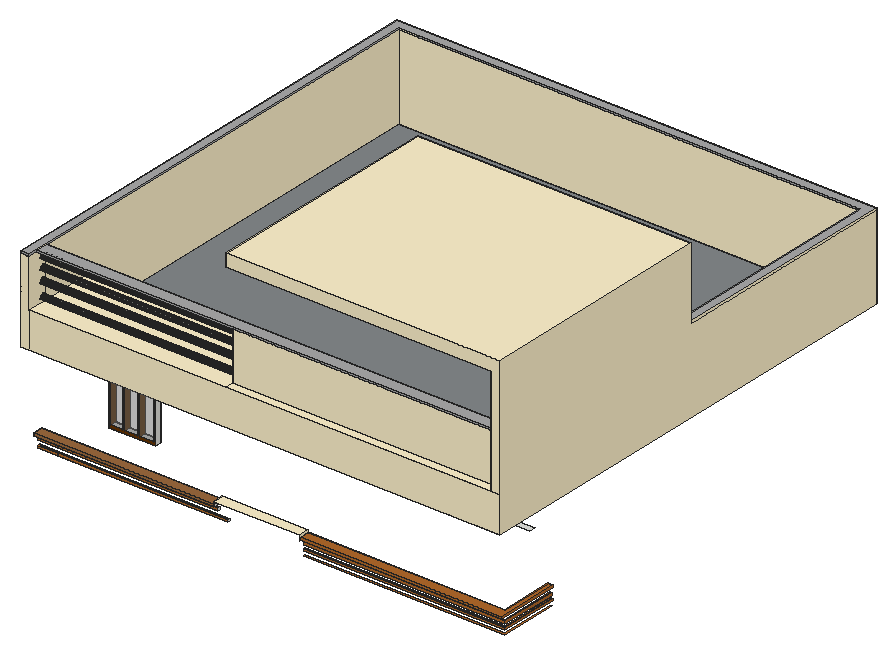
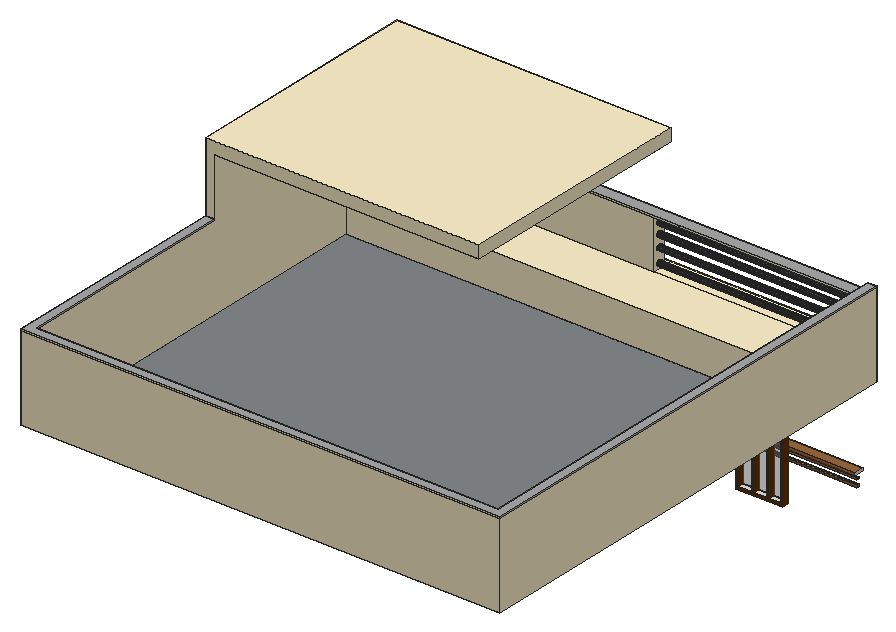
# SketchUp Ruby script. Lengths in inches.
U = 1.inch
M = Sketchup.active_model
def pt(a) = Geom::Point3d.new(a.map { |v| v * U })
def face(e, loops, mat)
  f = e.add_face(loops[0].map { |a| pt(a) })
  loops[1..].each { |l| e.add_face(l.map { |a| pt(a) }).erase! }
  f.material = f.back_material = mat if mat
  f
end
# faces: each face lists its corners as indices into pts; further lists are holes
def faces(e, pts, list, mat = nil) = list.each { |f| face(e, (f[0].is_a?(Array) ? f : [f]).map { |l| l.map { |i| pts[i] } }, mat) }
# xy, xz, yz: faces in a plane at the given z, y or x. An outline is a flat list of corners, or four numbers for a rectangle; further outlines are holes
def ring(l) = l.size == 4 ? [[l[0], l[1]], [l[2], l[1]], [l[2], l[3]], [l[0], l[3]]] : l.each_slice(2).to_a
def flat(e, list, mat, &to3) = list.each { |f| face(e, (f[0].is_a?(Array) ? f : [f]).map { |l| ring(l).map { |u, v| to3.(u, v) } }, mat) }
def xy(e, z, list, mat = nil) = flat(e, list, mat) { |x, y| [x, y, z] }
def xz(e, y, list, mat = nil) = flat(e, list, mat) { |x, z| [x, y, z] }
def yz(e, x, list, mat = nil) = flat(e, list, mat) { |y, z| [x, y, z] }
def lines(e, pts, list) = list.each { |a, b| e.add_line(pt(pts[a]), pt(pts[b])) }
# prism: a flat outline (further loops are holes) pulled along v
def prism(e, loops, v, mat = nil)
  f = face(e, loops, mat); d = Geom::Vector3d.new(v.map { |x| x * U })
  f.pushpull(f.normal.samedirection?(d) ? d.length : -d.length)
end
def box(e, o, s, mat = nil) = prism(e, [[o, [o[0] + s[0], o[1], o[2]], [o[0] + s[0], o[1] + s[1], o[2]], [o[0], o[1] + s[1], o[2]]]], [0, 0, s[2]], mat)
def at(x, y, z, deg = 0) = Geom::Transformation.translation(pt([x, y, z])) * Geom::Transformation.rotation(ORIGIN, Z_AXIS, deg.degrees)
def axes(o, x, y, z) = Geom::Transformation.new([*x, 0, *y, 0, *z, 0, *pt(o).to_a, 1])
def part(name) = M.definitions.add(name)
# library, detail: a bought-in or finely detailed component or shape, given as its bounding box
def library(name, o, s) = part(name).tap { |d| box(d.entities, o, s) }
def detail(e, o, s) = box(e.add_group.entities, o, s)
def put(e, d, t, mat = nil) = e.add_instance(d, t).tap { |i| i.material = mat if mat }
def group(e, t, mat = nil) = e.add_group.tap { |g| g.transformation = t; g.material = mat if mat }.entities
root = M.entities
M.materials.add("[Blacktop Old 01]").color = [132, 136, 139]
M.materials.add("[Brick Tumbled]").color = [135, 132, 132]
M.materials.add("[Color C08]").color = [102, 51, 0]
M.materials.add("[Color D01]").color = [255, 242, 204]
M.materials.add("[Color M03]").color = [170, 170, 170]
M.materials.add("[Metal Seamed]").color = [118, 119, 115]
M.materials.add("[Translucent Glass Gray]").color = [128, 128, 128]
M.materials["[Translucent Glass Gray]"].alpha = 0.5
M.materials.add("[Wood Bamboo]").color = [177, 105, 43]
M.materials.add("[Wood Floor]").color = [155, 105, 61]
xy(root,456.24,[[274.98,145.89,477.01,145.89,477.01,204.4,475.1875,204.4,475.1875,148.02,274.98,148.02]],"[Wood Bamboo]")
xy(root,459.55,[[9,146.02,28.82,148.14]])
xy(root,459.55,[[28.82,146.02,199.2,148.14]],"[Wood Bamboo]")
xy(root,460.3,[[274.98,145.89,274.98,148.02,475.1875,148.02,475.1875,205.64,477.01,205.64,477.01,145.89]],"[Wood Bamboo]")
xy(root,460.62,[[33.82,204.4,80.13,210.4]])
xy(root,461.67,[[9,146.02,28.82,148.14],[28.82,146.02,199.2,148.14]],"[Wood Bamboo]")
xy(root,462.43,[[274.98,145.89,477.01,145.89,477.01,205.64,475.1875,205.64,475.1875,148.02,274.98,148.02]],"[Wood Bamboo]")
xy(root,465.86,[[274.98,145.89,274.98,148.02,475.1875,148.02,475.1875,204.36,477.01,204.36,477.01,145.89]],"[Wood Bamboo]")
xy(root,466.42,[[9,146.02,28.82,148.14]])
xy(root,466.42,[[28.82,146.02,189.2,148.14]],"[Wood Bamboo]")
xy(root,468.36,[[274.98,145.89,477.01,145.89,477.01,204.36,475.1875,204.36,475.1875,148.02,274.98,148.02]],"[Wood Bamboo]")
xy(root,468.55,[[9,146.02,28.82,148.14],[28.82,146.02,189.2,148.14]],"[Wood Bamboo]")
xy(root,471.875,[[309.7,143.88,313.07,150.13]])
xy(root,472.05,[[[8.16,141.71,188.91,151.78],[68.13,143.88,71.51,150.13],[110.26,143.88,113.63,150.13]],[[274.98,141.71,274.98,151.78,472.375,151.78,472.375,205.65,477.34,205.65,477.34,141.71],[421.51,143.88,424.88,150.13]]],"[Wood Bamboo]")
xy(root,472.0625,[[472.3125,168.86,477.25,172.24]])
xy(root,472.3125,[[152.95,143.88,156.32,150.13]])
xy(root,472.4375,[[362.95,143.88,366.32,150.13]])
xy(root,472.875,[[25.45,143.88,28.82,150.13]])
xy(root,474.59,[[274.98,141.71,477.34,141.71,477.34,205.65,472.375,205.65,472.375,151.78,274.98,151.78]],"[Wood Bamboo]")
xy(root,474.59,[[8.16,141.71,188.91,151.78]],"[Wood Floor]")
xy(root,476.8125,[[188.91,140.9,274.98,151.78]],"[Color D01]")
xy(root,515.8125,[[108.75,204.4,156.75,210.4],[407.0625,204.4,455.0625,210.4]])
xy(root,526.43,[[33.82,204.4,80.13,210.4]])
xy(root,526.73,[[322.9,204.4,382.78,210.4]])
xy(root,551.8125,[[9,210.4,471,597.75]],"[Blacktop Old 01]")
xy(root,551.8125,[[172.75,192.4,292.75,204.4]],"[Brick Tumbled]")
xy(root,551.8125,[[[0,135.4,0,606.75,480,606.75,480,204.4,9,204.4,9,135.4],[9,210.4,471,597.75]],[9,135.4,172.75,204.4],[172.75,135.4,292.75,192.4],[292.75,135.4,480,204.4]],"[Color D01]")
xy(root,551.8125,[[11.75,154.17,19.6875,160.61],[27.8125,154.17,35,160.61],[43.5625,154.17,50.1875,160.61]],"[Wood Floor]")
xy(root,587.8125,[[9,135.4,205.99,156.62],[205.99,135.4,471,144.15],[205.99,144.15,471,156.62],[9,156.62,471,210.4]],"[Color D01]")
xy(root,635.8125,[[0,135.4,9,156.62],[9,144.15,205.99,156.62],[205.99,144.15,471,156.62],[0,156.62,0,606.75,480,606.75,480,375.16,471,375.16,471,597.75,9,597.75,9,156.62]],"[Color D01]")
xy(root,637.8125,[[0,135.4,9,135.4,9,597.75,471,597.75,471,375.16,480,375.16,480,606.75,0,606.75],[9,144.15,471,156.62]],"[Color M03]")
xy(root,695.23,[[205.99,135.4,471,375.16]],"[Color D01]")
xy(root,707.8125,[[205.99,135.4,480,375.16]],"[Color D01]")
xz(root,135.4,[[0,551.8125,9,635.8125],[9,551.8125,480,587.8125],[471,587.8125,480,587.8125,480,707.8125,205.99,707.8125,205.99,695.23,471,695.23]],"[Color D01]")
xz(root,135.4,[[0,635.8125,9,637.8125]],"[Color M03]")
xz(root,141.71,[[274.98,472.05,477.34,474.59]],"[Wood Bamboo]")
xz(root,141.71,[[8.16,472.05,188.91,474.59]],"[Wood Floor]")
xz(root,144.15,[[205.99,587.8125,471,635.8125]],"[Color D01]")
xz(root,144.15,[[9,635.8125,471,637.8125]],"[Color M03]")
xz(root,145.89,[[274.98,460.3,477.01,462.43],[274.98,465.86,477.01,468.36]],"[Wood Bamboo]")
xz(root,146.02,[[9,459.55,28.82,461.67],[28.82,459.55,199.2,461.67],[9,466.42,28.82,468.55],[28.82,466.42,189.2,468.55]],"[Wood Bamboo]")
xz(root,148.02,[[274.98,460.3,475.1875,462.43],[274.98,465.86,475.1875,468.36]],"[Wood Bamboo]")
xz(root,148.14,[[9,459.55,28.82,461.67],[28.82,459.55,199.2,461.67],[9,466.42,28.82,468.55],[28.82,466.42,189.2,468.55]],"[Wood Bamboo]")
xz(root,151.78,[[8.16,472.05,188.91,474.59],[274.98,472.05,472.375,474.59]],"[Wood Bamboo]")
xz(root,156.62,[[205.99,587.8125,471,635.8125],[9,635.8125,471,637.8125]],"[Color D01]")
xz(root,204.36,[[475.1875,465.86,477.01,468.36]])
xz(root,205.64,[[475.1875,460.3,477.01,462.43]])
xz(root,205.65,[[472.375,472.05,477.34,474.59]])
xz(root,210.4,[[9,551.8125,471,587.8125]],"[Color D01]")
xz(root,375.16,[[471,635.8125,480,637.8125],[471,637.8125,471,695.23,205.99,695.23,205.99,707.8125,480,707.8125,480,637.8125]],"[Color D01]")
xz(root,597.75,[[9,551.8125,471,635.8125],[9,635.8125,29.375,637.8125]],"[Color D01]")
xz(root,597.75,[[29.375,635.8125,471,637.8125]],"[Color M03]")
xz(root,606.75,[[0,551.8125,480,635.8125],[0,635.8125,480,637.8125]],"[Color D01]")
yz(root,0,[[135.4,551.8125,606.75,635.8125]],"[Color D01]")
yz(root,0,[[135.4,635.8125,606.75,637.8125]],"[Color M03]")
yz(root,8.16,[[141.71,472.05,151.78,474.59]])
yz(root,8.61,[[150.89,590.66,150.21,590.78,149.59,591.07,149.07,591.51,148.68,592.08,148.45,592.72,148.39,593.4,148.51,594.08,148.8,594.7,149.24,595.22,149.81,595.61,150.45,595.85,151.13,595.9,151.81,595.78,152.43,595.49,152.95,595.05,153.34,594.49,153.58,593.84,153.63,593.16,153.51,592.48,153.22,591.86,152.78,591.34,152.22,590.95,151.57,590.72]],"[Color D01]")
yz(root,9,[[210.4,551.8125,597.75,551.8125,597.75,635.8125,156.62,635.8125,156.62,587.8125,210.4,587.8125],[[135.4,587.8125,156.62,635.8125],[150.89,627.41,150.21,627.53,149.59,627.82,149.07,628.26,148.68,628.83,148.45,629.47,148.39,630.15,148.51,630.83,148.8,631.45,149.24,631.97,149.81,632.36,150.45,632.6,151.13,632.65,151.81,632.53,152.43,632.24,152.95,631.8,153.34,631.24,153.58,630.59,153.63,629.91,153.51,629.23,153.22,628.61,152.78,628.09,152.22,627.7,151.57,627.47],[150.89,616.85,150.21,616.97,149.59,617.26,149.07,617.7,148.68,618.26,148.45,618.91,148.39,619.59,148.51,620.27,148.8,620.89,149.24,621.41,149.81,621.8,150.45,622.03,151.13,622.09,151.81,621.97,152.43,621.68,152.95,621.24,153.34,620.67,153.58,620.03,153.63,619.35,153.51,618.67,153.22,618.05,152.78,617.53,152.22,617.14,151.57,616.9]],[144.15,635.8125,156.62,637.8125]],"[Color D01]")
yz(root,9,[[135.4,635.8125,144.15,637.8125],[156.62,635.8125,597.75,637.8125]],"[Color M03]")
yz(root,9.17,[[150.89,604.85,150.21,604.97,149.59,605.26,149.07,605.7,148.68,606.26,148.45,606.91,148.39,607.59,148.51,608.27,148.8,608.89,149.24,609.41,149.81,609.8,150.45,610.03,151.13,610.09,151.81,609.97,152.43,609.68,152.95,609.24,153.34,608.67,153.58,608.03,153.63,607.35,153.51,606.67,153.22,606.05,152.78,605.53,152.22,605.14,151.57,604.9]],"[Color D01]")
yz(root,28.82,[[146.02,459.55,148.14,461.67],[146.02,466.42,148.14,468.55]])
yz(root,33.82,[[204.4,460.62,210.4,526.43]])
yz(root,80.13,[[204.4,460.62,210.4,526.43]])
yz(root,188.91,[[141.71,472.05,151.78,474.59]])
yz(root,188.91,[[140.9,472.05,141.71,474.59],[140.9,474.59,151.78,476.8125]],"[Color D01]")
yz(root,189.2,[[146.02,466.42,148.14,468.55]])
yz(root,199.2,[[146.02,459.55,148.14,461.67]])
yz(root,205.99,[[[144.15,587.8125,156.62,635.8125],[150.89,627.41,151.57,627.47,152.22,627.7,152.78,628.09,153.22,628.61,153.51,629.23,153.63,629.91,153.58,630.59,153.34,631.24,152.95,631.8,152.43,632.24,151.81,632.53,151.13,632.65,150.45,632.6,149.81,632.36,149.24,631.97,148.8,631.45,148.51,630.83,148.39,630.15,148.45,629.47,148.68,628.83,149.07,628.26,149.59,627.82,150.21,627.53],[150.89,616.85,151.57,616.9,152.22,617.14,152.78,617.53,153.22,618.05,153.51,618.67,153.63,619.35,153.58,620.03,153.34,620.67,152.95,621.24,152.43,621.68,151.81,621.97,151.13,622.09,150.45,622.03,149.81,621.8,149.24,621.41,148.8,620.89,148.51,620.27,148.39,619.59,148.45,618.91,148.68,618.26,149.07,617.7,149.59,617.26,150.21,616.97],[150.89,604.85,151.57,604.9,152.22,605.14,152.78,605.53,153.22,606.05,153.51,606.67,153.63,607.35,153.58,608.03,153.34,608.67,152.95,609.24,152.43,609.68,151.81,609.97,151.13,610.09,150.45,610.03,149.81,609.8,149.24,609.41,148.8,608.89,148.51,608.27,148.39,607.59,148.45,606.91,148.68,606.26,149.07,605.7,149.59,605.26,150.21,604.97],[150.89,590.66,151.57,590.72,152.22,590.95,152.78,591.34,153.22,591.86,153.51,592.48,153.63,593.16,153.58,593.84,153.34,594.49,152.95,595.05,152.43,595.49,151.81,595.78,151.13,595.9,150.45,595.85,149.81,595.61,149.24,595.22,148.8,594.7,148.51,594.08,148.39,593.4,148.45,592.72,148.68,592.08,149.07,591.51,149.59,591.07,150.21,590.78]],[135.4,695.23,375.16,707.8125]],"[Color D01]")
yz(root,274.98,[[141.71,472.05,151.78,474.59]])
yz(root,274.98,[[140.9,472.05,141.71,474.59],[140.9,474.59,151.78,476.8125]],"[Color D01]")
yz(root,471,[[210.4,551.8125,210.4,587.8125,156.62,587.8125,156.62,637.8125,135.4,637.8125,135.4,695.23,375.16,695.23,375.16,635.8125,597.75,635.8125,597.75,551.8125],[135.4,587.8125,144.15,635.8125],[144.15,587.8125,156.62,635.8125],[135.4,635.8125,144.15,637.8125],[144.15,635.8125,156.62,637.8125]],"[Color D01]")
yz(root,471,[[375.16,635.8125,597.75,637.8125]],"[Color M03]")
yz(root,472.375,[[151.78,472.05,205.65,474.59]],"[Wood Bamboo]")
yz(root,475.1875,[[148.02,460.3,205.64,462.43],[148.02,465.86,204.36,468.36]],"[Wood Bamboo]")
yz(root,477.01,[[145.89,460.3,205.64,462.43],[145.89,465.86,204.36,468.36]],"[Wood Bamboo]")
yz(root,477.34,[[141.71,472.05,205.65,474.59]],"[Wood Bamboo]")
yz(root,480,[[135.4,551.8125,606.75,551.8125,606.75,635.8125,375.16,635.8125,375.16,707.8125,135.4,707.8125],[375.16,635.8125,606.75,637.8125]],"[Color D01]")
p = [[205.99,150.89,590.66],[205.99,150.21,590.78],[8.61,150.21,590.78],[8.61,150.89,590.66],[205.99,151.57,590.72],[8.61,151.57,590.72],
  [205.99,152.22,590.95],[8.61,152.22,590.95],[205.99,149.59,591.07],[8.61,149.59,591.07],[205.99,152.78,591.34],[8.61,152.78,591.34],
  [205.99,149.07,591.51],[8.61,149.07,591.51],[205.99,153.22,591.86],[8.61,153.22,591.86],[205.99,148.68,592.08],[8.61,148.68,592.08],
  [205.99,153.51,592.48],[8.61,153.51,592.48],[205.99,148.45,592.72],[8.61,148.45,592.72],[205.99,153.63,593.16],[8.61,153.63,593.16],
  [205.99,148.39,593.4],[8.61,148.39,593.4],[205.99,153.58,593.84],[8.61,153.58,593.84],[205.99,148.51,594.08],[8.61,148.51,594.08],
  [205.99,153.34,594.49],[8.61,153.34,594.49],[205.99,148.8,594.7],[8.61,148.8,594.7],[205.99,152.95,595.05],[8.61,152.95,595.05],
  [205.99,149.24,595.22],[8.61,149.24,595.22],[205.99,152.43,595.49],[8.61,152.43,595.49],[205.99,149.81,595.61],[8.61,149.81,595.61],
  [205.99,151.81,595.78],[8.61,151.81,595.78],[205.99,150.45,595.85],[8.61,150.45,595.85],[205.99,151.13,595.9],[8.61,151.13,595.9],
  [205.99,150.89,604.85],[205.99,150.21,604.97],[9.17,150.21,604.97],[9.17,150.89,604.85],[205.99,151.57,604.9],[9.17,151.57,604.9],
  [205.99,152.22,605.14],[9.17,152.22,605.14],[205.99,149.59,605.26],[9.17,149.59,605.26],[205.99,152.78,605.53],[9.17,152.78,605.53],
  [205.99,149.07,605.7],[9.17,149.07,605.7],[205.99,153.22,606.05],[9.17,153.22,606.05],[205.99,148.68,606.26],[9.17,148.68,606.26],
  [205.99,153.51,606.67],[9.17,153.51,606.67],[205.99,148.45,606.91],[9.17,148.45,606.91],[205.99,153.63,607.35],[9.17,153.63,607.35],
  [205.99,148.39,607.59],[9.17,148.39,607.59],[205.99,153.58,608.03],[9.17,153.58,608.03],[205.99,148.51,608.27],[9.17,148.51,608.27],
  [205.99,153.34,608.67],[9.17,153.34,608.67],[205.99,148.8,608.89],[9.17,148.8,608.89],[205.99,152.95,609.24],[9.17,152.95,609.24],
  [205.99,149.24,609.41],[9.17,149.24,609.41],[205.99,152.43,609.68],[9.17,152.43,609.68],[205.99,149.81,609.8],[9.17,149.81,609.8],
  [205.99,151.81,609.97],[9.17,151.81,609.97],[205.99,150.45,610.03],[9.17,150.45,610.03],[205.99,151.13,610.09],[9.17,151.13,610.09],
  [205.99,150.89,616.85],[205.99,150.21,616.97],[9,150.21,616.97],[9,150.89,616.85],[205.99,151.57,616.9],[9,151.57,616.9],
  [205.99,152.22,617.14],[9,152.22,617.14],[205.99,149.59,617.26],[9,149.59,617.26],[205.99,152.78,617.53],[9,152.78,617.53],
  [205.99,149.07,617.7],[9,149.07,617.7],[205.99,153.22,618.05],[9,153.22,618.05],[205.99,148.68,618.26],[9,148.68,618.26],
  [205.99,153.51,618.67],[9,153.51,618.67],[205.99,148.45,618.91],[9,148.45,618.91],[205.99,153.63,619.35],[9,153.63,619.35],
  [205.99,148.39,619.59],[9,148.39,619.59],[205.99,153.58,620.03],[9,153.58,620.03],[205.99,148.51,620.27],[9,148.51,620.27],
  [205.99,153.34,620.67],[9,153.34,620.67],[205.99,148.8,620.89],[9,148.8,620.89],[205.99,152.95,621.24],[9,152.95,621.24],
  [205.99,149.24,621.41],[9,149.24,621.41],[205.99,152.43,621.68],[9,152.43,621.68],[205.99,149.81,621.8],[9,149.81,621.8],
  [205.99,151.81,621.97],[9,151.81,621.97],[205.99,150.45,622.03],[9,150.45,622.03],[205.99,151.13,622.09],[9,151.13,622.09],
  [205.99,150.89,627.41],[205.99,150.21,627.53],[9,150.21,627.53],[9,150.89,627.41],[205.99,151.57,627.47],[9,151.57,627.47],
  [205.99,149.59,627.82],[9,149.59,627.82],[205.99,152.22,627.7],[9,152.22,627.7],[205.99,152.78,628.09],[9,152.78,628.09],
  [205.99,149.07,628.26],[9,149.07,628.26],[205.99,153.22,628.61],[9,153.22,628.61],[205.99,148.68,628.83],[9,148.68,628.83],
  [205.99,153.51,629.23],[9,153.51,629.23],[205.99,148.45,629.47],[9,148.45,629.47],[205.99,153.63,629.91],[9,153.63,629.91],
  [205.99,148.39,630.15],[9,148.39,630.15],[205.99,153.58,630.59],[9,153.58,630.59],[205.99,148.51,630.83],[9,148.51,630.83],
  [205.99,153.34,631.24],[9,153.34,631.24],[205.99,148.8,631.45],[9,148.8,631.45],[205.99,152.95,631.8],[9,152.95,631.8],
  [205.99,149.24,631.97],[9,149.24,631.97],[205.99,152.43,632.24],[9,152.43,632.24],[205.99,149.81,632.36],[9,149.81,632.36],
  [205.99,151.81,632.53],[9,151.81,632.53],[205.99,150.45,632.6],[9,150.45,632.6],[205.99,151.13,632.65],[9,151.13,632.65]]
faces(root,p,[[0,1,2,3],[4,0,3,5],[6,4,5,7],[1,8,9,2],[10,6,7,11],[8,12,13,9],[14,10,11,15],[12,16,17,13],
  [18,14,15,19],[16,20,21,17],[22,18,19,23],[20,24,25,21],[26,22,23,27],[24,28,29,25],[30,26,27,31],[28,32,33,29],
  [34,30,31,35],[32,36,37,33],[38,34,35,39],[36,40,41,37],[42,38,39,43],[40,44,45,41],[44,46,47,45],[46,42,43,47],
  [48,49,50,51],[52,48,51,53],[54,52,53,55],[49,56,57,50],[58,54,55,59],[56,60,61,57],[62,58,59,63],[60,64,65,61],
  [66,62,63,67],[64,68,69,65],[70,66,67,71],[68,72,73,69],[74,70,71,75],[72,76,77,73],[78,74,75,79],[76,80,81,77],
  [82,78,79,83],[80,84,85,81],[86,82,83,87],[84,88,89,85],[90,86,87,91],[88,92,93,89],[92,94,95,93],[94,90,91,95],
  [96,97,98,99],[100,96,99,101],[102,100,101,103],[97,104,105,98],[106,102,103,107],[104,108,109,105],[110,106,107,111],[108,112,113,109],
  [114,110,111,115],[112,116,117,113],[118,114,115,119],[116,120,121,117],[122,118,119,123],[120,124,125,121],[126,122,123,127],[124,128,129,125],
  [130,126,127,131],[128,132,133,129],[134,130,131,135],[132,136,137,133],[138,134,135,139],[136,140,141,137],[140,142,143,141],[142,138,139,143],
  [144,145,146,147],[148,144,147,149],[145,150,151,146],[152,148,149,153],[154,152,153,155],[150,156,157,151],[158,154,155,159],[156,160,161,157],
  [162,158,159,163],[160,164,165,161],[166,162,163,167],[164,168,169,165],[170,166,167,171],[168,172,173,169],[174,170,171,175],[172,176,177,173],
  [178,174,175,179],[176,180,181,177],[182,178,179,183],[180,184,185,181],[186,182,183,187],[184,188,189,185],[190,186,187,191],[188,190,191,189]],"[Metal Seamed]")
g1 = group(root,at(33.75,204.4,460.62))
xy(g1,0,[[0,0,46.38,6.12]],"[Color C08]")
xy(g1,2.88,[[2.03,0,13.84,6.12],[15.61,0,28.92,6.12],[30.6875,0,44.35,6.12]])
xy(g1,62.93,[[2.03,0,13.84,6.12],[15.61,0,28.92,6.12],[30.6875,0,44.35,6.12]],"[Color C08]")
xy(g1,65.8125,[[0,0,46.38,6.12]],"[Color C08]")
xz(g1,0,[[[0,0,46.38,65.8125],[30.6875,2.88,44.35,62.93],[15.61,2.88,28.92,62.93],[2.03,2.88,13.84,62.93]]],"[Color C08]")
xz(g1,0,[[2.03,2.88,13.84,62.93],[15.61,2.88,28.92,62.93],[30.6875,2.88,44.35,62.93]],"[Translucent Glass Gray]")
xz(g1,6.12,[[[0,0,46.38,65.8125],[30.6875,2.88,44.35,62.93],[15.61,2.88,28.92,62.93],[2.03,2.88,13.84,62.93]]],"[Color C08]")
yz(g1,0,[[0,0,6.12,65.8125]],"[Color C08]")
yz(g1,2.03,[[0,2.88,6.12,62.93]],"[Color C08]")
yz(g1,13.84,[[0,2.88,6.12,62.93]],"[Color C08]")
yz(g1,15.61,[[0,2.88,6.12,62.93]],"[Color C08]")
yz(g1,28.92,[[0,2.88,6.12,62.93]],"[Color C08]")
yz(g1,30.6875,[[0,2.88,6.12,62.93]],"[Color C08]")
yz(g1,44.35,[[0,2.88,6.12,62.93]],"[Color C08]")
yz(g1,46.38,[[0,0,6.12,65.8125]],"[Color C08]")
